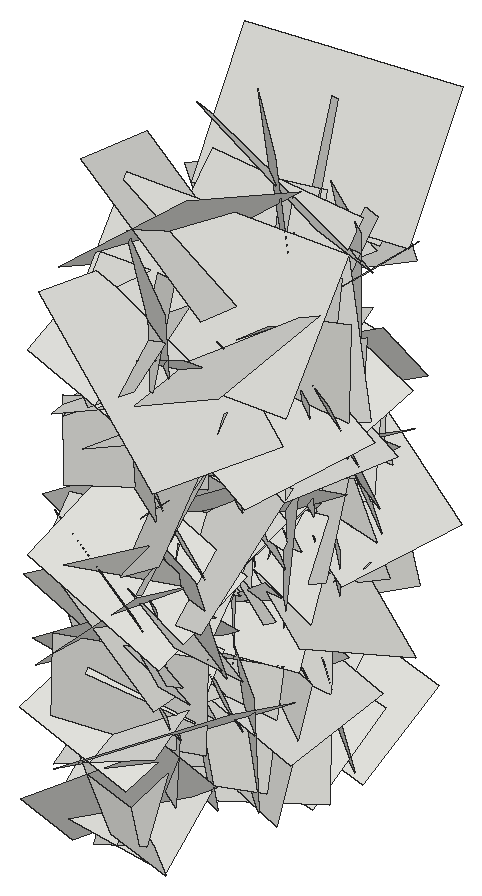
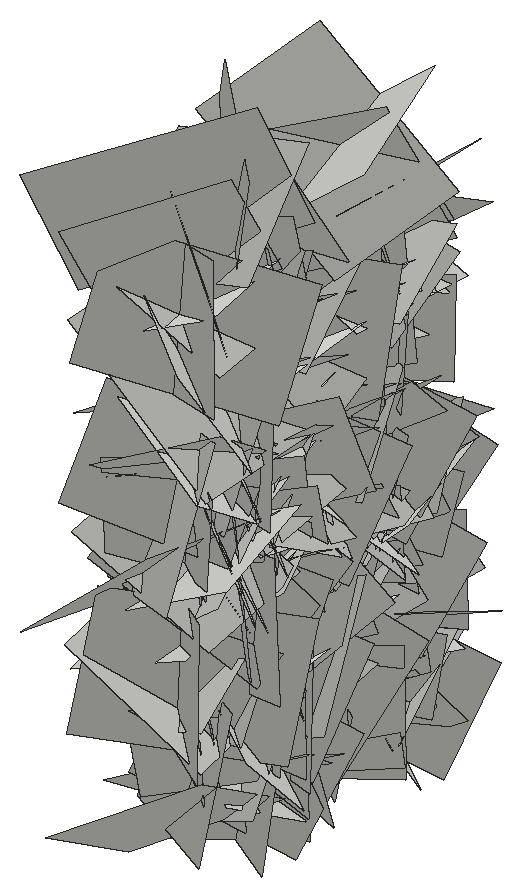
# SketchUp Ruby script. Lengths in inches.
U = 1.inch
M = Sketchup.active_model
def pt(a) = Geom::Point3d.new(a.map { |v| v * U })
def face(e, loops, mat)
  f = e.add_face(loops[0].map { |a| pt(a) })
  loops[1..].each { |l| e.add_face(l.map { |a| pt(a) }).erase! }
  f.material = f.back_material = mat if mat
  f
end
# faces: each face lists its corners as indices into pts; further lists are holes
def faces(e, pts, list, mat = nil) = list.each { |f| face(e, (f[0].is_a?(Array) ? f : [f]).map { |l| l.map { |i| pts[i] } }, mat) }
# xy, xz, yz: faces in a plane at the given z, y or x. An outline is a flat list of corners, or four numbers for a rectangle; further outlines are holes
def ring(l) = l.size == 4 ? [[l[0], l[1]], [l[2], l[1]], [l[2], l[3]], [l[0], l[3]]] : l.each_slice(2).to_a
def flat(e, list, mat, &to3) = list.each { |f| face(e, (f[0].is_a?(Array) ? f : [f]).map { |l| ring(l).map { |u, v| to3.(u, v) } }, mat) }
def xy(e, z, list, mat = nil) = flat(e, list, mat) { |x, y| [x, y, z] }
def xz(e, y, list, mat = nil) = flat(e, list, mat) { |x, z| [x, y, z] }
def yz(e, x, list, mat = nil) = flat(e, list, mat) { |y, z| [x, y, z] }
def lines(e, pts, list) = list.each { |a, b| e.add_line(pt(pts[a]), pt(pts[b])) }
# prism: a flat outline (further loops are holes) pulled along v
def prism(e, loops, v, mat = nil)
  f = face(e, loops, mat); d = Geom::Vector3d.new(v.map { |x| x * U })
  f.pushpull(f.normal.samedirection?(d) ? d.length : -d.length)
end
def box(e, o, s, mat = nil) = prism(e, [[o, [o[0] + s[0], o[1], o[2]], [o[0] + s[0], o[1] + s[1], o[2]], [o[0], o[1] + s[1], o[2]]]], [0, 0, s[2]], mat)
def at(x, y, z, deg = 0) = Geom::Transformation.translation(pt([x, y, z])) * Geom::Transformation.rotation(ORIGIN, Z_AXIS, deg.degrees)
def axes(o, x, y, z) = Geom::Transformation.new([*x, 0, *y, 0, *z, 0, *pt(o).to_a, 1])
def part(name) = M.definitions.add(name)
# library, detail: a bought-in or finely detailed component or shape, given as its bounding box
def library(name, o, s) = part(name).tap { |d| box(d.entities, o, s) }
def detail(e, o, s) = box(e.add_group.entities, o, s)
def put(e, d, t, mat = nil) = e.add_instance(d, t).tap { |i| i.material = mat if mat }
def group(e, t, mat = nil) = e.add_group.tap { |g| g.transformation = t; g.material = mat if mat }.entities
root = M.entities
c1 = part("Component\#6")
p = [[0.01,0,0],[0,3.24,4.54],[4.32,3.24,4.54],[4.33,0,0]]
faces(c1.entities,p,[[0,1,2,3]])
put(root,c1,axes([38.11,158.45,22.43],[0.19892,0.24365,-1.12098],[-0.08242,-1.13056,-0.25875],[-1.21318,0.11676,-0.16622]))
put(root,c1,axes([34.14,151.13,9.12],[-0.15296,0.67587,0.31221],[0.03502,0.32352,-0.68509],[0.78839,0.11676,0.09101]))
put(root,c1,axes([38.11,148.76,4.0625],[-0.10183,-0.75916,-0.2873],[-0.20096,-0.26032,0.75126],[-0.83661,0.15493,-0.14549]))
put(root,c1,axes([38.11,155.05,20.66],[-0.11898,0.43702,0.87755],[0.10329,0.88388,-0.42771],[-1.03402,0.038,-0.1437]))
put(root,c1,axes([38.11,154.79,8.7],[0.06507,0.61236,-0.89404],[0.03144,-0.89608,-0.61173],[-1.14823,0.01016,-0.06741]))
put(root,c1,axes([34.14,151.99,2.12],[-0.1775,0.68354,0.35821],[0.06031,0.37649,-0.69181],[0.81579,0.12089,0.12909]))
put(root,c1,axes([34.14,151.79,4.27],[-0.00282,-0.67031,0.14172],[-0.04158,0.14164,0.66918],[0.72504,0.00552,0.03892]))
put(root,c1,axes([34.14,147.62,1.41],[-0.08717,-0.06025,0.7019],[0.04865,0.70471,0.06586],[0.74517,-0.05306,0.07781]))
put(root,c1,axes([34.14,156.87,7.65],[0.00449,0.50233,-0.39291],[0.02578,-0.39276,-0.50188],[0.67552,0.01165,0.02176]))
put(root,c1,axes([34.14,153.92,20.8125],[0.01755,0.277,-0.54123],[0.05617,-0.54003,-0.27476],[0.64202,0.03967,0.03883]))
put(root,c1,axes([38.11,152.6,3.91],[-0.02426,0.68313,0.69515],[0.0107,0.69547,-0.68312],[-1.03305,-0.00884,-0.0234]))
put(root,c1,axes([34.14,147.13,6.96],[-0.04816,-0.19283,0.63159],[0.07038,0.62854,0.19668],[0.69645,-0.07685,0.0238]))
put(root,c1,axes([38.11,158.68,8.63],[0.07829,-0.94373,0.27717],[-0.10215,0.26967,0.94388],[-1.03759,-0.09775,-0.07202]))
put(root,c1,axes([38.11,152.91,14.99],[0.05042,0.65822,-0.8803],[0.11398,-0.87969,-0.65195],[-1.15954,-0.05785,-0.10236]))
put(root,c1,axes([38.11,159.16,9.85],[0.13765,0.1916,-1.18129],[0.14512,-1.1828,-0.17679],[-1.2602,-0.11528,-0.14939]))
put(root,c1,axes([38.11,157.06,14.03],[0.04606,-0.47436,-0.98882],[0.12961,-0.98133,0.47614],[-1.15527,-0.12901,0.01399]))
put(root,c1,axes([38.11,149.64,15.49],[0.05397,-0.71515,0.49033],[-0.26351,0.45852,0.69456],[-0.88054,-0.18105,-0.1778]))
put(root,c1,axes([34.14,148.39,13.69],[0.056,0.56116,0.2115],[0.06403,0.20626,-0.56234],[0.63244,-0.07057,0.03821]))
put(root,c1,axes([38.11,147.71,9.53],[0.0202,0.73421,-0.62443],[-0.01239,-0.62433,-0.73445],[-1.02159,0.02209,-0.00344]))
put(root,c1,axes([34.14,146.72,8.375],[0.05548,0.31048,0.67068],[-0.12303,0.66747,-0.29994],[0.77368,0.08387,-0.09579]))
put(root,c1,axes([38.11,152.28,1.18],[0.22482,-0.75958,0.923],[0.06114,0.94282,0.76264],[-1.2656,-0.08938,0.2008]))
put(root,c1,axes([38.11,154.73,4.99],[0.23466,-0.21907,1.02966],[-0.17179,1.03255,0.25453],[-1.10257,-0.20751,0.17949]))
put(root,c1,axes([34.14,148.44,10.1],[0.02371,0.59128,0.15103],[0.13632,0.14317,-0.57956],[0.63236,-0.05303,0.11928]))
put(root,c1,axes([34.14,154.81,5.31],[0.03271,-0.68931,-0.29186],[-0.0897,-0.29345,0.68411],[0.78838,-0.00479,0.08995]))
put(root,c1,axes([34.14,155.07,5.6],[-0.26442,-0.95782,0.42161],[-0.12666,0.45666,0.96674],[1.10204,-0.17733,0.21227]))
put(root,c1,axes([38.11,146.38,17.95],[-0.09245,0.38694,0.78979],[0.04684,0.79459,-0.38441],[-0.93107,0.00155,-0.09776]))
put(root,c1,axes([34.14,155.43,2.74],[0.05213,0.12024,0.7107],[-0.06472,0.71048,-0.11598],[0.7613,0.05216,-0.05853]))
put(root,c1,axes([38.11,149.03,14.67],[0.12882,0.64149,-0.81464],[-0.00451,-0.8199,-0.64626],[-1.09909,0.07855,-0.09282]))
put(root,c1,axes([34.14,145.53,10.42],[-0.22479,1.04725,-0.16356],[-0.16331,-0.19548,-1.05191],[1.11161,0.18306,-0.18761]))
put(root,c1,axes([38.11,147.21,13.43],[0.06341,1.09172,0.23851],[0.19798,0.22572,-1.08003],[-1.16785,0.09755,-0.17015]))
put(root,c1,axes([34.14,146.09,12.1875],[-0.18427,0.52878,-0.65011],[0.11203,-0.64482,-0.55274],[0.8812,0.19255,-0.06567]))
put(root,c1,axes([38.11,151.57,3.27],[-0.14157,0.02397,-0.74069],[-0.04702,-0.75154,-0.01632],[-0.78414,0.04073,0.1347]))
put(root,c1,axes([34.14,154.48,3.89],[0.11783,0.23417,0.69133],[-0.11259,0.69704,-0.21902],[0.76547,0.06648,-0.13863]))
put(root,c1,axes([34.14,152.53,7.1875],[0.08757,-0.64703,0.3684],[-0.09594,0.35919,0.65114],[0.78338,0.11632,0.03856]))
put(root,c1,axes([38.11,153.68,-0.24],[-0.08313,-0.05331,0.78078],[-0.05564,0.78328,0.04821],[-0.82769,-0.0473,-0.08166]))
put(root,c1,axes([34.14,155.23,10.47],[-0.04155,0.12694,-0.87349],[-0.11983,-0.86787,-0.12105],[0.92792,-0.10639,-0.05475]))
put(root,c1,axes([38.11,154.93,13.48],[0.13332,0.92748,-0.67904],[0.1887,-0.69057,-0.91025],[-1.20375,-0.00553,-0.2179]))
put(root,c1,axes([38.11,152.46,19.1],[0.24316,-1.11668,0.32256],[0.08367,0.34299,1.13127],[-1.22923,-0.19755,0.14081]))
put(root,c1,axes([38.11,149.625,17.57],[-0.05592,-0.7816,-0.40589],[0.0657,-0.4089,0.77935],[-0.93124,0.01809,0.07936]))
put(root,c1,axes([34.14,153.02,6.56],[0.04835,0.51462,-0.41299],[0.10228,-0.41473,-0.50612],[0.69191,0.02534,0.10368]))
put(root,c1,axes([34.14,155.74,21.65],[-0.00825,-0.17983,-0.66547],[0.14401,-0.65286,0.17483],[0.71636,0.12918,-0.04281]))
put(root,c1,axes([38.11,147.06,-0.97],[-0.01135,-0.66277,0.66685],[0.09721,0.66298,0.66039],[-0.99185,0.07256,0.05709]))
put(root,c1,axes([34.14,154.86,6.54],[-0.11481,0.21277,-0.79232],[0.09254,-0.79167,-0.22453],[0.86468,0.11298,-0.08117]))
put(root,c1,axes([38.11,155.95,10.68],[-0.04823,-0.00518,0.84226],[0.02844,0.84305,0.00663],[-0.89236,0.02715,-0.04531]))
put(root,c1,axes([38.11,146.53,12.92],[-0.03124,-0.05121,0.8385],[0.00373,0.839,0.05136],[-0.89046,0.00531,-0.0292]))
put(root,c1,axes([38.11,152.8,10.75],[0.04843,-0.82009,-0.82841],[0.32646,-0.79109,0.80013],[-1.19171,-0.25004,0.18553]))
put(root,c1,axes([34.14,155.82,10.86],[-0.10869,-0.77244,0.23734],[0.13092,0.22145,0.77409],[0.8465,-0.13343,-0.08925]))
put(root,c1,axes([34.14,156.49,11.61],[-0.16435,-0.92659,-0.48849],[-0.14398,-0.47186,0.93815],[1.10094,-0.20004,0.04977]))
put(root,c1,axes([38.11,153.88,7.81],[-0.12498,-0.19712,-0.75186],[0.05107,-0.76085,0.19192],[-0.82232,-0.01729,0.12619]))
put(root,c1,axes([34.14,154.72,7.86],[0.01434,-0.12328,-0.7123],[0.10241,-0.70572,0.12398],[0.75939,0.0975,-0.00327]))
put(root,c1,axes([38.11,155.22,14.18],[0.0107,0.67836,0.43703],[-0.08223,0.43585,-0.67474],[-0.8514,-0.03357,0.07066]))
put(root,c1,axes([34.14,152.55,8.85],[-0.17208,0.39932,0.93109],[-0.08126,0.93542,-0.41455],[1.07081,0.13515,0.11817]))
put(root,c1,axes([38.11,155.14,21.07],[0.01676,0.7943,-0.14622],[-0.08914,-0.14383,-0.79043],[-0.85145,0.03069,0.07988]))
put(root,c1,axes([34.14,158.76,13.54],[-0.17018,-0.33172,-0.9968],[-0.1229,-0.99662,0.35033],[1.10678,-0.16167,-0.11436]))
put(root,c1,axes([38.11,151.77,10.3],[-0.00621,-0.04081,-0.81439],[-0.02737,-0.814,0.04098],[-0.86391,0.02608,0.00455]))
put(root,c1,axes([38.11,149.67,1.32],[-0.10197,-0.47157,-0.58691],[0.00963,-0.59236,0.47447],[-0.798,0.05311,0.08072]))
put(root,c1,axes([34.14,154.27,5.56],[-0.10843,0.64197,-0.78685],[-0.13439,-0.79271,-0.63027],[1.06801,-0.03458,-0.15919]))
put(root,c1,axes([38.11,154.27,5.56],[0.10843,0.64197,-0.78685],[0.13439,-0.79271,-0.63027],[-1.06801,-0.03458,-0.15919]))
put(root,c1,axes([34.14,149.67,1.32],[0.10197,-0.47157,-0.58691],[-0.00963,-0.59236,0.47447],[0.798,0.05311,0.08072]))
put(root,c1,axes([34.14,151.77,10.3],[0.00621,-0.04081,-0.81439],[0.02737,-0.814,0.04098],[0.86391,0.02608,0.00455]))
put(root,c1,axes([38.11,158.76,13.54],[0.17018,-0.33172,-0.9968],[0.1229,-0.99662,0.35033],[-1.10678,-0.16167,-0.11436]))
put(root,c1,axes([34.14,155.14,21.07],[-0.01676,0.7943,-0.14622],[0.08914,-0.14383,-0.79043],[0.85145,0.03069,0.07988]))
put(root,c1,axes([38.11,152.55,8.85],[0.17208,0.39932,0.93109],[0.08126,0.93542,-0.41455],[-1.07081,0.13515,0.11817]))
put(root,c1,axes([34.14,155.22,14.18],[-0.0107,0.67836,0.43703],[0.08223,0.43585,-0.67474],[0.8514,-0.03357,0.07066]))
put(root,c1,axes([38.11,154.72,7.86],[-0.01434,-0.12328,-0.7123],[-0.10241,-0.70572,0.12398],[-0.75939,0.0975,-0.00327]))
put(root,c1,axes([34.14,153.88,7.81],[0.12498,-0.19712,-0.75186],[-0.05107,-0.76085,0.19192],[0.82232,-0.01729,0.12619]))
put(root,c1,axes([38.11,156.49,11.61],[0.16435,-0.92659,-0.48849],[0.14398,-0.47186,0.93815],[-1.10094,-0.20004,0.04977]))
put(root,c1,axes([38.11,155.82,10.86],[0.10869,-0.77244,0.23734],[-0.13092,0.22145,0.77409],[-0.8465,-0.13343,-0.08925]))
put(root,c1,axes([34.14,152.8,10.75],[-0.04843,-0.82009,-0.82841],[-0.32646,-0.79109,0.80013],[1.19171,-0.25004,0.18553]))
put(root,c1,axes([34.14,146.53,12.92],[0.03124,-0.05121,0.8385],[-0.00373,0.839,0.05136],[0.89046,0.00531,-0.0292]))
put(root,c1,axes([34.14,155.95,10.68],[0.04823,-0.00518,0.84226],[-0.02844,0.84305,0.00663],[0.89236,0.02715,-0.04531]))
put(root,c1,axes([38.11,154.86,6.54],[0.11481,0.21277,-0.79232],[-0.09254,-0.79167,-0.22453],[-0.86468,0.11298,-0.08117]))
put(root,c1,axes([34.14,147.06,-0.97],[0.01135,-0.66277,0.66685],[-0.09721,0.66298,0.66039],[0.99185,0.07256,0.05709]))
put(root,c1,axes([38.11,155.74,21.65],[0.00825,-0.17983,-0.66547],[-0.14401,-0.65286,0.17483],[-0.71636,0.12918,-0.04281]))
put(root,c1,axes([38.11,153.02,6.56],[-0.04835,0.51462,-0.41299],[-0.10228,-0.41473,-0.50612],[-0.69191,0.02534,0.10368]))
put(root,c1,axes([34.14,149.625,17.57],[0.05592,-0.7816,-0.40589],[-0.0657,-0.4089,0.77935],[0.93124,0.01809,0.07936]))
put(root,c1,axes([34.14,152.46,19.1],[-0.24316,-1.11668,0.32256],[-0.08367,0.34299,1.13127],[1.22923,-0.19755,0.14081]))
put(root,c1,axes([34.14,154.93,13.48],[-0.13332,0.92748,-0.67904],[-0.1887,-0.69057,-0.91025],[1.20375,-0.00553,-0.2179]))
put(root,c1,axes([38.11,155.23,10.47],[0.04155,0.12694,-0.87349],[0.11983,-0.86787,-0.12105],[-0.92792,-0.10639,-0.05475]))
put(root,c1,axes([34.14,153.68,-0.24],[0.08313,-0.05331,0.78078],[0.05564,0.78328,0.04821],[0.82769,-0.0473,-0.08166]))
put(root,c1,axes([38.11,152.53,7.1875],[-0.08757,-0.64703,0.3684],[0.09594,0.35919,0.65114],[-0.78338,0.11632,0.03856]))
put(root,c1,axes([38.11,154.48,3.89],[-0.11783,0.23417,0.69133],[0.11259,0.69704,-0.21902],[-0.76547,0.06648,-0.13863]))
put(root,c1,axes([34.14,151.57,3.27],[0.14157,0.02397,-0.74069],[0.04702,-0.75154,-0.01632],[0.78414,0.04073,0.1347]))
put(root,c1,axes([38.11,146.09,12.1875],[0.18427,0.52878,-0.65011],[-0.11203,-0.64482,-0.55274],[-0.8812,0.19255,-0.06567]))
put(root,c1,axes([34.14,147.21,13.43],[-0.06341,1.09172,0.23851],[-0.19798,0.22572,-1.08003],[1.16785,0.09755,-0.17015]))
put(root,c1,axes([38.11,145.53,10.42],[0.22479,1.04725,-0.16356],[0.16331,-0.19548,-1.05191],[-1.11161,0.18306,-0.18761]))
put(root,c1,axes([34.14,149.03,14.67],[-0.12882,0.64149,-0.81464],[0.00451,-0.8199,-0.64626],[1.09909,0.07855,-0.09282]))
put(root,c1,axes([38.11,155.43,2.74],[-0.05213,0.12024,0.7107],[0.06472,0.71048,-0.11598],[-0.7613,0.05216,-0.05853]))
put(root,c1,axes([34.14,146.38,17.95],[0.09245,0.38694,0.78979],[-0.04684,0.79459,-0.38441],[0.93107,0.00155,-0.09776]))
put(root,c1,axes([38.11,155.07,5.6],[0.26442,-0.95782,0.42161],[0.12666,0.45666,0.96674],[-1.10204,-0.17733,0.21227]))
put(root,c1,axes([38.11,154.81,5.31],[-0.03271,-0.68931,-0.29186],[0.0897,-0.29345,0.68411],[-0.78838,-0.00479,0.08995]))
put(root,c1,axes([38.11,148.44,10.1],[-0.02371,0.59128,0.15103],[-0.13632,0.14317,-0.57956],[-0.63236,-0.05303,0.11928]))
put(root,c1,axes([34.14,154.73,4.99],[-0.23466,-0.21907,1.02966],[0.17179,1.03255,0.25453],[1.10257,-0.20751,0.17949]))
put(root,c1,axes([34.14,152.28,1.18],[-0.22482,-0.75958,0.923],[-0.06114,0.94282,0.76264],[1.2656,-0.08938,0.2008]))
put(root,c1,axes([38.11,146.72,8.375],[-0.05548,0.31048,0.67068],[0.12303,0.66747,-0.29994],[-0.77368,0.08387,-0.09579]))
put(root,c1,axes([34.14,147.71,9.53],[-0.0202,0.73421,-0.62443],[0.01239,-0.62433,-0.73445],[1.02159,0.02209,-0.00344]))
put(root,c1,axes([38.11,148.39,13.69],[-0.056,0.56116,0.2115],[-0.06403,0.20626,-0.56234],[-0.63244,-0.07057,0.03821]))
put(root,c1,axes([34.14,149.64,15.49],[-0.05397,-0.71515,0.49033],[0.26351,0.45852,0.69456],[0.88054,-0.18105,-0.1778]))
put(root,c1,axes([34.14,157.06,14.03],[-0.04606,-0.47436,-0.98882],[-0.12961,-0.98133,0.47614],[1.15527,-0.12901,0.01399]))
put(root,c1,axes([34.14,159.16,9.85],[-0.13765,0.1916,-1.18129],[-0.14512,-1.1828,-0.17679],[1.2602,-0.11528,-0.14939]))
put(root,c1,axes([34.14,152.91,14.99],[-0.05042,0.65822,-0.8803],[-0.11398,-0.87969,-0.65195],[1.15954,-0.05785,-0.10236]))
put(root,c1,axes([34.14,158.68,8.63],[-0.07829,-0.94373,0.27717],[0.10215,0.26967,0.94388],[1.03759,-0.09775,-0.07202]))
put(root,c1,axes([38.11,147.13,6.96],[0.04816,-0.19283,0.63159],[-0.07038,0.62854,0.19668],[-0.69645,-0.07685,0.0238]))
put(root,c1,axes([34.14,152.6,3.91],[0.02426,0.68313,0.69515],[-0.0107,0.69547,-0.68312],[1.03305,-0.00884,-0.0234]))
put(root,c1,axes([38.11,153.92,20.8125],[-0.01755,0.277,-0.54123],[-0.05617,-0.54003,-0.27476],[-0.64202,0.03967,0.03883]))
put(root,c1,axes([38.11,156.87,7.65],[-0.00449,0.50233,-0.39291],[-0.02578,-0.39276,-0.50188],[-0.67552,0.01165,0.02176]))
put(root,c1,axes([38.11,147.62,1.41],[0.08717,-0.06025,0.7019],[-0.04865,0.70471,0.06586],[-0.74517,-0.05306,0.07781]))
put(root,c1,axes([38.11,151.79,4.27],[0.00282,-0.67031,0.14172],[0.04158,0.14164,0.66918],[-0.72504,0.00552,0.03892]))
put(root,c1,axes([38.11,151.99,2.12],[0.1775,0.68354,0.35821],[-0.06031,0.37649,-0.69181],[-0.81579,0.12089,0.12909]))
put(root,c1,axes([34.14,154.79,8.7],[-0.06507,0.61236,-0.89404],[-0.03144,-0.89608,-0.61173],[1.14823,0.01016,-0.06741]))
put(root,c1,axes([34.14,155.05,20.66],[0.11898,0.43702,0.87755],[-0.10329,0.88388,-0.42771],[1.03402,0.038,-0.1437]))
put(root,c1,axes([34.14,148.76,4.0625],[0.10183,-0.75916,-0.2873],[0.20096,-0.26032,0.75126],[0.83661,0.15493,-0.14549]))
put(root,c1,axes([38.11,151.13,9.12],[0.15296,0.67587,0.31221],[-0.03502,0.32352,-0.68509],[-0.78839,0.11676,0.09101]))
put(root,c1,axes([34.14,158.45,22.43],[-0.19892,0.24365,-1.12098],[0.08242,-1.13056,-0.25875],[1.21318,0.11676,-0.16622]))
put(root,c1,axes([34.14,153.47,7.93],[-0.25077,0.36385,-1.26635],[-0.08689,-1.28818,-0.35481],[1.39394,-0.01484,-0.24993]))
put(root,c1,axes([38.11,151.91,13.09],[0.06029,-0.61389,0.14039],[-0.0496,0.13645,0.61563],[-0.66568,-0.06576,-0.03315]))
put(root,c1,axes([38.11,155.37,8.05],[0.03179,-0.04018,0.69029],[0.07893,0.6871,0.03676],[-0.72868,0.07267,0.03409]))
put(root,c1,axes([38.11,147.25,18.09],[0.11506,-0.20062,0.68841],[0.02156,0.69683,0.19986],[-0.75976,-0.01061,0.10993]))
put(root,c1,axes([38.11,146,16.15],[0.10062,0.63244,0.10884],[-0.07256,0.11937,-0.63396],[-0.67636,0.08128,0.0842]))
put(root,c1,axes([34.14,157.74,11.21],[0.0595,-0.6331,0.72554],[0.06262,0.72766,0.63038],[1.01877,-0.00775,-0.08112]))
put(root,c1,axes([34.14,160.22,19.0625],[-0.13961,-0.68099,-1.03193],[-0.07146,-1.03227,0.68982],[1.30861,-0.12902,-0.07242]))
put(root,c1,axes([38.11,149.02,5.32],[0.19432,-0.67994,0.40742],[0.04988,0.42677,0.69106],[-0.83874,-0.13215,0.13549]))
put(root,c1,axes([34.14,154.9,1.8],[0.03269,0.90387,0.50014],[0.00572,0.50021,-0.90434],[1.09498,-0.0296,-0.01021]))
put(root,c1,axes([38.11,152.72,13.34],[0.14332,-0.62648,-0.12325],[-0.10799,-0.14554,0.62801],[-0.66813,-0.11086,-0.12794]))
put(root,c1,axes([34.14,157.43,12.97],[-0.1074,-0.05602,-1.35571],[-0.22854,-1.34155,0.07155],[1.42001,-0.22014,-0.09102]))
put(root,c1,axes([34.14,151.01,19.39],[0.01021,0.65154,-0.69294],[0.23408,-0.67557,-0.63214],[0.98066,0.15447,0.1581]))
put(root,c1,axes([34.14,148.31,17.26],[0.09379,0.98835,0.28145],[-0.01751,0.28383,-0.99149],[1.08916,-0.08054,-0.04018]))
put(root,c1,axes([34.14,155.4,17.52],[-0.19723,0.3027,-1.19403],[0.0763,-1.20284,-0.31615],[1.30348,0.11621,-0.16216]))
put(root,c1,axes([34.14,145.87,3.84],[0.08046,-0.07863,0.91675],[0.19442,0.90269,0.06223],[0.95574,-0.17701,-0.08983]))
put(root,c1,axes([34.14,148.09,7.11],[-0.15706,0.67864,1.02073],[0.03183,1.02986,-0.68036],[1.29889,0.05683,0.1401]))
put(root,c1,axes([34.14,148.93,-0.125],[-0.17085,0.2332,1.25619],[-0.02467,1.2654,-0.2379],[1.35409,0.05247,0.15416]))
put(root,c1,axes([34.14,158.83,13.98],[0.00743,-1.2386,0.03478],[-0.17851,0.0335,1.22715],[1.30124,0.01167,0.16814]))
put(root,c1,axes([34.14,152.08,1.74],[0.04493,0.85391,0.54577],[0.09586,0.54089,-0.85328],[1.06994,-0.08432,0.05353]))
put(root,c1,axes([34.14,151.75,19.45],[0.16935,0.44212,0.83371],[0.05466,0.84022,-0.45546],[0.99881,-0.12095,-0.11643]))
put(root,c1,axes([38.11,150.18,6.375],[0.17639,-0.58204,-0.33942],[-0.00316,-0.35025,0.59915],[-0.71419,-0.1422,-0.08648]))
put(root,c1,axes([38.11,148.65,3.04],[0.12439,-0.47488,0.46679],[0.05284,0.47892,0.47469],[-0.70386,-0.04797,0.11813]))
put(root,c1,axes([34.14,156.6875,24.44],[0.16473,0.01802,-1.18121],[-0.23771,-1.16927,-0.04735],[1.22945,-0.22849,0.14911]))
put(root,c1,axes([34.14,147.43,1.76],[0.0449,0.15818,1.07958],[0.0304,1.07985,-0.15935],[1.15617,-0.03454,-0.03773]))
put(root,c1,axes([34.14,158.38,15.93],[-0.03304,0.59909,-1.16183],[-0.1621,-1.15585,-0.5919],[1.37611,-0.12177,-0.09762]))
put(root,c1,axes([34.14,156.09,10.89],[0.02844,-1.01096,-0.23497],[0.17327,-0.228,0.99963],[1.08645,0.06282,-0.15327]))
put(root,c1,axes([34.14,159.05,4.5],[0.22831,-0.97739,-0.02602],[-0.01319,-0.02938,1.00067],[1.03632,0.21495,0.01847]))
put(root,c1,axes([34.14,157.5,5.99],[0.02733,0.34478,-1.12821],[-0.04378,-1.12752,-0.34552],[1.24973,-0.04704,0.01257]))
put(root,c1,axes([34.14,147.25,11.15],[0.01251,0.83252,-0.66438],[0.16644,-0.65852,-0.82239],[1.1167,0.08883,0.13002]))
put(root,c1,axes([34.14,153.16,13.74],[0.07693,-1.07175,0.44962],[-0.07215,0.4458,1.07364],[1.22986,0.09319,0.03486]))
put(root,c1,axes([34.14,150.33,13.2],[-0.24126,0.02501,1.36725],[0.05252,1.3853,-0.01709],[1.44858,-0.04606,0.22834]))
put(root,c1,axes([34.14,144.59,11.1],[0.20686,0.83944,0.54314],[0.00436,0.55271,-0.85571],[1.05982,-0.16612,-0.10249]))
put(root,c1,axes([34.14,153.72,24.55],[-0.10736,0.8301,-0.78481],[0.26067,-0.75358,-0.8288],[1.18252,0.24148,0.11144]))
put(root,c1,axes([34.14,148.8125,12.02],[0.02959,0.36254,-1.01381],[0.21176,-0.99828,-0.35148],[1.12146,0.17893,0.09312]))
put(root,c1,axes([34.14,148.37,14.37],[0.13394,0.02599,1.3483],[-0.3112,1.32226,0.00203],[1.39518,0.29244,-0.12899]))
put(root,c1,axes([34.14,151.84,12.71],[0.09641,-0.969,-0.91768],[-0.24854,-0.9171,0.94515],[1.39265,-0.09659,0.2322]))
put(root,c1,axes([34.14,152.41,8.09],[-0.02535,-1.06677,0.60381],[0.0625,0.60222,1.06631],[1.29785,-0.04984,-0.03955]))
put(root,c1,axes([34.14,153.41,21.56],[0.04666,0.60871,1.19242],[-0.17987,1.18598,-0.59916],[1.40769,0.13136,-0.11609]))
put(root,c1,axes([34.14,154.4,5.48],[-0.14525,-0.2612,-1.20099],[0.27145,-1.18798,0.22915],[1.27422,0.2233,-0.18571]))
put(root,c1,axes([34.14,153.21,11.43],[-0.14123,-0.96535,-0.93141],[0.15435,-0.94087,0.95433],[1.41351,0.00629,-0.19727]))
put(root,c1,axes([34.14,157.09,9.16],[0.26081,-0.66319,-0.77037],[0.09697,-0.77495,0.69635],[1.07312,0.23121,0.12431]))
put(root,c1,axes([34.14,149.27,6.59],[-0.15688,1.33929,-0.00269],[0.18956,0.01708,-1.33541],[1.40693,0.14704,0.17962]))
put(root,c1,axes([34.14,149.82,11.51],[0.16938,-0.10345,1.35904],[-0.25816,1.34416,0.13095],[1.4215,0.25644,-0.13816]))
put(root,c1,axes([34.14,155.16,12.125],[0.20792,1.23942,0.0793],[-0.14973,0.10203,-1.24521],[1.30793,-0.18535,-0.15516]))
put(root,c1,axes([34.14,151.77,16.16],[0.14743,1.12249,0.38129],[0.0578,0.37744,-1.13105],[1.25528,-0.14922,0.00729]))
put(root,c1,axes([34.14,145.22,20.96],[0.20751,1.35949,-0.09859],[-0.20583,-0.07077,-1.36145],[1.43011,-0.20745,-0.18164]))
put(root,c1,axes([34.14,149.47,1.18],[0.22795,-1.08393,0.44752],[0.03192,0.45993,1.09954],[1.24263,0.18702,-0.11034]))
put(root,c1,axes([34.14,155.15,17.37],[0.02517,0.60882,-1.16754],[0.2041,-1.15679,-0.59929],[1.38075,0.1599,0.10987]))
put(root,c1,axes([34.14,146.56,18.67],[0.08115,0.67304,1.19325],[0.03541,1.19384,-0.67552],[1.45175,-0.06674,-0.05023]))
put(root,c1,axes([34.14,150.46,17.01],[0.04698,1.34267,-0.16756],[0.13374,-0.17102,-1.33703],[1.42802,-0.02815,0.13073]))
put(root,c1,axes([34.14,150.02,13.53],[0.11354,-0.10924,1.28227],[0.18202,1.27641,0.09439],[1.35193,-0.16268,-0.1204]))
put(root,c1,axes([34.14,153.54,10.59],[0.17173,1.22834,-0.55665],[0.01226,-0.5619,-1.23655],[1.42944,-0.14275,0.07748]))
put(root,c1,axes([34.14,151.36,16.73],[0.05564,-1.33407,-0.12972],[0.26745,-0.11766,1.31218],[1.39538,0.07575,-0.24633]))
put(root,c1,axes([34.14,148.21,18.05],[0.18781,1.38239,0.05917],[0.11095,0.04609,-1.39025],[1.46247,-0.18102,0.09787]))
